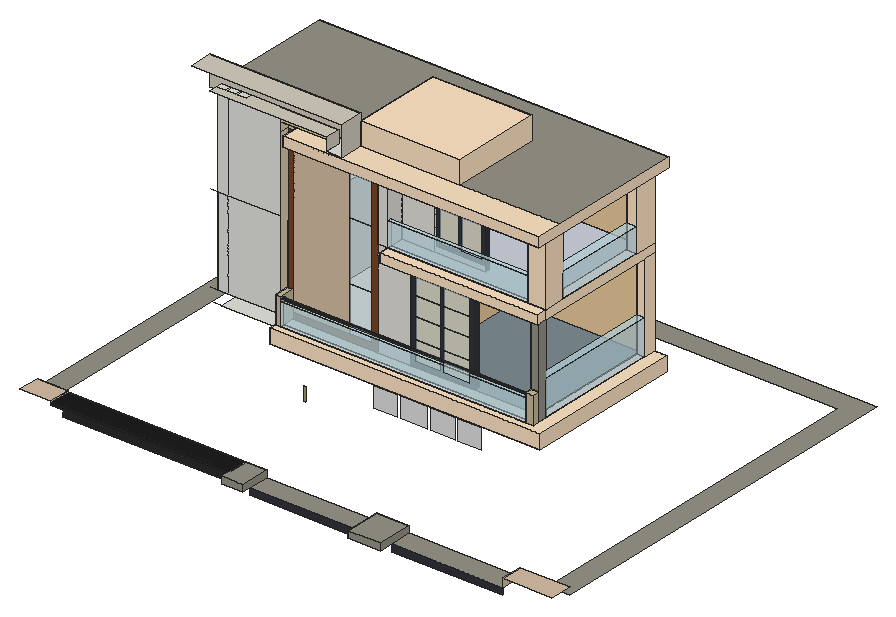
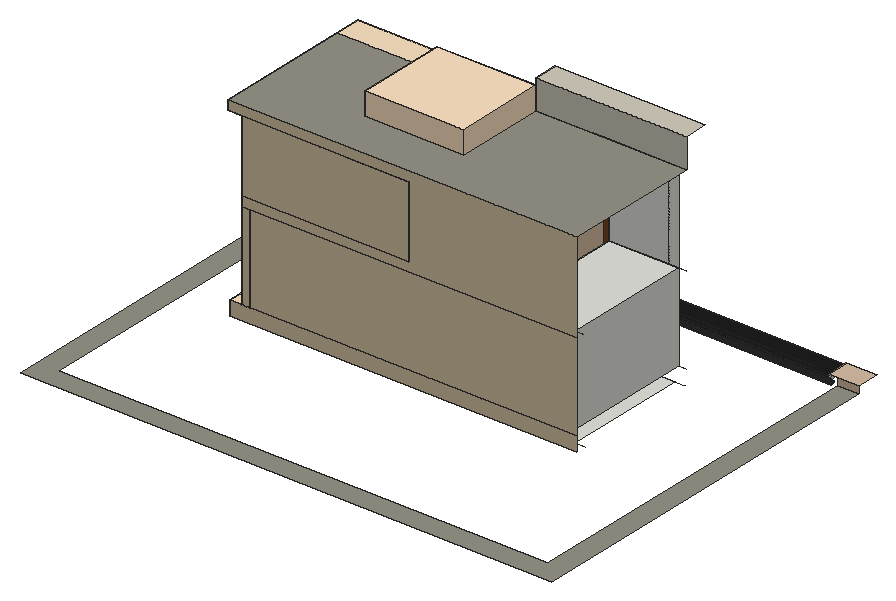
# SketchUp Ruby script. Lengths in inches.
U = 1.inch
M = Sketchup.active_model
def pt(a) = Geom::Point3d.new(a.map { |v| v * U })
def face(e, loops, mat)
  f = e.add_face(loops[0].map { |a| pt(a) })
  loops[1..].each { |l| e.add_face(l.map { |a| pt(a) }).erase! }
  f.material = f.back_material = mat if mat
  f
end
# faces: each face lists its corners as indices into pts; further lists are holes
def faces(e, pts, list, mat = nil) = list.each { |f| face(e, (f[0].is_a?(Array) ? f : [f]).map { |l| l.map { |i| pts[i] } }, mat) }
# xy, xz, yz: faces in a plane at the given z, y or x. An outline is a flat list of corners, or four numbers for a rectangle; further outlines are holes
def ring(l) = l.size == 4 ? [[l[0], l[1]], [l[2], l[1]], [l[2], l[3]], [l[0], l[3]]] : l.each_slice(2).to_a
def flat(e, list, mat, &to3) = list.each { |f| face(e, (f[0].is_a?(Array) ? f : [f]).map { |l| ring(l).map { |u, v| to3.(u, v) } }, mat) }
def xy(e, z, list, mat = nil) = flat(e, list, mat) { |x, y| [x, y, z] }
def xz(e, y, list, mat = nil) = flat(e, list, mat) { |x, z| [x, y, z] }
def yz(e, x, list, mat = nil) = flat(e, list, mat) { |y, z| [x, y, z] }
def lines(e, pts, list) = list.each { |a, b| e.add_line(pt(pts[a]), pt(pts[b])) }
# prism: a flat outline (further loops are holes) pulled along v
def prism(e, loops, v, mat = nil)
  f = face(e, loops, mat); d = Geom::Vector3d.new(v.map { |x| x * U })
  f.pushpull(f.normal.samedirection?(d) ? d.length : -d.length)
end
def box(e, o, s, mat = nil) = prism(e, [[o, [o[0] + s[0], o[1], o[2]], [o[0] + s[0], o[1] + s[1], o[2]], [o[0], o[1] + s[1], o[2]]]], [0, 0, s[2]], mat)
def at(x, y, z, deg = 0) = Geom::Transformation.translation(pt([x, y, z])) * Geom::Transformation.rotation(ORIGIN, Z_AXIS, deg.degrees)
def axes(o, x, y, z) = Geom::Transformation.new([*x, 0, *y, 0, *z, 0, *pt(o).to_a, 1])
def part(name) = M.definitions.add(name)
# library, detail: a bought-in or finely detailed component or shape, given as its bounding box
def library(name, o, s) = part(name).tap { |d| box(d.entities, o, s) }
def detail(e, o, s) = box(e.add_group.entities, o, s)
def put(e, d, t, mat = nil) = e.add_instance(d, t).tap { |i| i.material = mat if mat }
def group(e, t, mat = nil) = e.add_group.tap { |g| g.transformation = t; g.material = mat if mat }.entities
root = M.entities
M.materials.add("[0012_Bisque]").color = [252, 225, 194]
M.materials.add("[0012_Bisque]1").color = [255, 228, 196]
M.materials.add("[0035_Tan]").color = [234, 201, 156]
M.materials.add("[Color M08]").color = [30, 30, 30]
M.materials.add("[Concrete Pavers Block Multi]").color = [124, 140, 145]
M.materials.add("[Field Square Tile]").color = [217, 201, 169]
M.materials.add("[Formica Graystone]").color = [209, 204, 189]
M.materials.add("[Formica Graystone]1").color = [149, 146, 135]
M.materials.add("[Formica Laminate Dark]").color = [50, 53, 60]
M.materials.add("[Formica Laminate Light]").color = [213, 189, 164]
M.materials.add("[Marble Carrara Floor Tile]").color = [204, 208, 219]
M.materials.add("[Marble Carrara Gold Floor Tile]").color = [225, 223, 217]
M.materials.add("[Quartz Light Brown]").color = [199, 184, 152]
M.materials.add("[Translucent Glass Gray]").color = [128, 128, 128]
M.materials["[Translucent Glass Gray]"].alpha = 0.5
M.materials.add("[Translucent Glass Safety]").color = [204, 235, 244]
M.materials["[Translucent Glass Safety]"].alpha = 0.5
M.materials.add("[Wood Bamboo]").color = [177, 105, 43]
M.materials.add("[Wood Lumber ButtJoined]").color = [164, 152, 112]
M.materials.add("[Wood Veneer 01]").color = [120, 70, 37]
xy(root,70.6875,[[463.03,0,507.04,19.125],[284.59,8,312.84,19.125],[463.03,19.125,507.04,48.44]])
xy(root,70.6875,[[312.84,19.125,463.03,48.44],[507.04,19.125,658.96,48.44]],"[Formica Graystone]1")
xy(root,72,[[0,48.44,29.31,48.44,29.31,542.96,697.25,542.96,697.25,48.44,726.5625,48.44,726.5625,572.27,0,572.27]],"[Formica Graystone]1")
xy(root,76.75,[[153.57,19.125,161.5,27.41],[161.5,19.125,169.43,27.41],[41.54,27.41,48.35,37.79],[153.57,27.41,161.5,37.79],[161.5,27.41,169.43,37.79],
  [277.34,27.41,284.59,37.79],[153.57,37.79,161.5,48.44],[161.5,37.79,169.43,48.44]])
xy(root,76.75,[[41.54,19.125,41.54,27.41,48.35,27.41,48.35,37.79,41.54,37.79,41.54,48.44,153.57,48.44,153.57,19.125],[169.43,19.125,169.43,48.44,284.59,48.44,284.59,37.79,277.34,37.79,277.34,27.41,284.59,27.41,284.59,19.125]],"[Color M08]")
xy(root,79.91,[[41.54,19.125,284.59,48.44]],"[Color M08]")
xy(root,80,[[463.03,0,507.04,48.44],[284.59,8,312.84,48.44]],"[Formica Graystone]1")
xy(root,81.8125,[[0,19.125,41.54,48.44],[658.96,19.125,726.5625,48.44]],"[Formica Laminate Light]")
xy(root,118.13,[[320.36,216.4,477.43,230.18]])
xy(root,129,[[106.34,230.18,513.1,400.72],[513.1,230.18,526.89,414.5]])
xy(root,129,[[198.4375,197.31,567.07,216.4],[526.89,216.4,567.07,230.18],[526.89,230.18,567.07,414.5]],"[0012_Bisque]")
xy(root,148.25,[[198.4375,206.85,205.86,227.35],[205.86,206.85,539.81,211.77],[539.81,206.85,550.76,216.4],[205.86,211.77,539.81,227.35],[539.81,216.4,550.76,227.35],
  [103.52,227.35,198.4375,403.54],[198.4375,227.35,358.57,403.54],[358.57,227.35,367.31,403.54],[367.31,227.35,453.56,235.59],[539.81,227.35,550.76,396.98],
  [539.81,396.98,550.76,414.5]])
xy(root,148.25,[[198.4375,197.31,567.07,197.31,567.07,414.5,550.76,414.5,550.76,206.85,198.4375,206.85]],"[0012_Bisque]")
xy(root,148.25,[[453.56,227.35,539.81,227.35,539.81,403.54,367.31,403.54,367.31,235.59,453.56,235.59]],"[Concrete Pavers Block Multi]")
xy(root,178.125,[[205.86,206.85,539.81,211.77]],"[Translucent Glass Safety]")
xy(root,184.9375,[[198.4375,206.85,205.86,227.35],[539.81,206.85,550.76,216.4]],"[Quartz Light Brown]")
xy(root,196.25,[[539.81,227.35,550.76,396.98]],"[Translucent Glass Safety]")
xy(root,268.25,[[539.81,214.29,550.76,216.4],[539.81,216.4,550.76,227.35],[103.52,227.35,198.4375,403.54],[358.57,227.35,367.31,403.54],[367.31,227.35,453.56,235.59],
  [539.81,396.98,550.76,414.5],[198.4375,403.54,358.57,414.5],[358.57,403.54,367.31,414.5],[367.31,403.54,539.81,414.5]])
xy(root,268.25,[[335.01,214.29,539.81,227.35]],"[0012_Bisque]1")
xy(root,268.25,[[453.56,227.35,453.56,235.59,367.31,235.59,367.31,403.54,539.81,403.54,539.81,396.98,550.76,396.98,550.76,227.35]],"[Wood Bamboo]")
xy(root,280.9375,[[321.82,227.35,321.82,414.5,550.76,414.5,550.76,383,537.52,383,537.52,401.25,335.07,401.25,335.07,227.35],[335.07,227.35,526.35,233.16],[526.35,227.35,526.35,240.6,537.52,240.6,537.52,256.72,550.76,256.72,550.76,227.35],[335.07,251.53,449.88,256.72],[537.52,256.72,550.76,383]])
xy(root,280.9375,[[335.01,214.29,550.76,227.35]],"[0012_Bisque]1")
xy(root,280.9375,[[335.07,233.16,526.35,233.16,526.35,240.6,537.52,240.6,537.52,401.25,335.07,401.25,335.07,256.72,449.88,256.72,449.88,251.53,335.07,251.53]],"[Marble Carrara Floor Tile]")
xy(root,314.4375,[[335.07,227.35,526.35,233.16],[537.52,256.72,550.76,383]],"[Translucent Glass Safety]")
xy(root,379.375,[[321.82,227.35,321.82,414.5,550.76,414.5,550.76,383,537.52,383,537.52,401.25,335.07,401.25,335.07,227.35],[526.35,227.35,526.35,240.6,537.52,240.6,537.52,256.72,550.76,256.72,550.76,227.35],[335.07,251.53,449.88,256.72]])
xy(root,379.375,[[219.95,192.17,219.95,227.35,550.76,227.35,550.76,414.5,569.82,414.5,569.82,192.17]],"[0012_Bisque]1")
xy(root,379.375,[[335.07,227.35,335.07,251.53,449.88,251.53,449.88,256.72,335.07,256.72,335.07,401.25,537.52,401.25,537.52,383,550.76,383,550.76,256.72,537.52,256.72,537.52,240.6,526.35,240.6,526.35,227.35]],"[Wood Bamboo]")
xy(root,392.375,[[276.68,195.77,276.68,216.4,219.95,216.4,219.95,227.35,297.93,227.35,297.93,195.77],[198.4375,216.4,219.95,227.35],[297.93,227.35,433.12,350.92]])
xy(root,392.375,[[219.95,192.17,276.68,216.4],[276.68,192.17,297.93,195.77],[297.93,192.17,569.82,227.35]],"[0012_Bisque]")
xy(root,392.375,[[92.5625,227.35,297.93,227.35,297.93,350.92,433.12,350.92,433.12,227.35,569.82,227.35,569.82,414.5,92.5625,414.5]],"[Formica Graystone]1")
xy(root,409.95,[[117.23,208.71,128.74,216.4],[131.17,208.71,142.68,216.4],[145.54,208.71,157.05,216.4]])
xy(root,409.95,[[117.23,195.77,117.23,208.71,128.74,208.71,128.74,216.4,131.17,216.4,131.17,208.71,142.68,208.71,142.68,216.4,145.54,216.4,145.54,208.71,157.05,208.71,157.05,216.4,276.68,216.4,276.68,195.77]],"[Formica Graystone]")
xy(root,423.3125,[[297.93,227.35,433.12,350.92]],"[0012_Bisque]1")
xy(root,432.8125,[[92.5625,195.77,297.93,227.35]],"[Formica Graystone]")
xz(root,0,[[463.03,70.6875,507.04,80]],"[Formica Graystone]1")
xz(root,8,[[284.59,70.6875,312.84,80]],"[Formica Graystone]1")
xz(root,19.125,[[41.54,76.75,284.59,79.91]],"[Color M08]")
xz(root,19.125,[[507.04,61.39,658.96,70.6875],[312.84,61.83,463.03,70.6875]],"[Formica Laminate Dark]")
xz(root,48.44,[[41.54,76.75,284.59,79.91]],"[Color M08]")
xz(root,48.44,[[284.59,70.6875,312.84,80],[463.03,70.6875,507.04,80]],"[Formica Graystone]1")
xz(root,48.44,[[0,72,29.31,81.8125]],"[Formica Laminate Light]")
xz(root,192.17,[[219.95,379.375,569.82,392.375]],"[0012_Bisque]")
xz(root,197.31,[[198.4375,129,567.07,148.25]],"[0012_Bisque]")
xz(root,206.85,[[198.4375,148.25,205.86,184.9375],[539.81,148.25,550.76,184.9375]],"[Quartz Light Brown]")
xz(root,206.85,[[205.86,148.25,539.81,178.125]],"[Translucent Glass Safety]")
xz(root,211.77,[[205.86,148.25,539.81,178.125]],"[Translucent Glass Safety]")
xz(root,214.29,[[335.01,268.25,550.76,280.9375]],"[0012_Bisque]1")
xz(root,216.4,[[539.81,148.25,550.76,178.125],[539.81,178.125,550.76,184.9375]])
xz(root,216.4,[[198.4375,392.375,276.68,409.95]],"[Field Square Tile]")
xz(root,216.4,[[539.81,184.9375,550.76,268.25]],"[Formica Graystone]1")
xz(root,216.4,[[324.95,85.55,358.29,113.55],[361.76,85.55,398.73,113.55],[402.19,85.55,436.48,113.55],[439.94,85.55,472.85,113.55]],"[Translucent Glass Gray]")
xz(root,216.4,[[228.85,61.59,231.85,79.84]],"[Wood Lumber ButtJoined]")
xz(root,227.35,[[103.52,148.25,117.23,268.25],[117.23,148.25,198.4375,268.25],[198.4375,148.25,205.86,184.9375],[539.81,148.25,550.76,196.25],[103.52,268.25,117.23,392.375],
  [117.23,268.25,198.4375,392.375],[335.01,268.25,550.76,280.9375]])
xz(root,227.35,[[526.35,280.9375,550.76,379.375]],"[0012_Bisque]")
xz(root,227.35,[[297.93,392.375,433.12,423.3125]],"[0012_Bisque]1")
xz(root,227.35,[[198.4375,379.375,219.95,392.375]],"[Field Square Tile]")
xz(root,227.35,[[92.5625,392.375,297.93,432.8125]],"[Formica Graystone]")
xz(root,227.35,[[539.81,196.25,550.76,268.25]],"[Formica Graystone]1")
xz(root,227.35,[[[367.31,148.25,453.56,268.25],[373.52,154.46,447.35,262.04]],[407.96,154.46,412.12,262.04]],"[Formica Laminate Dark]")
xz(root,227.35,[[205.86,156.84,283.0625,156.84,283.0625,370.78,207.03,370.78,207.03,184.9375,205.86,184.9375]],"[Formica Laminate Light]")
xz(root,227.35,[[321.82,148.25,367.31,268.25],[321.82,268.25,335.01,280.9375],[321.82,280.9375,335.07,379.375]],"[Marble Carrara Gold Floor Tile]")
xz(root,227.35,[[373.52,154.46,407.96,182.08],[412.12,154.46,447.35,182.08],[283.0625,156.84,313.23,218.375],[373.52,182.08,407.96,209.7],[412.12,182.08,447.35,209.7],
  [373.52,209.7,407.96,236.15],[412.12,209.7,447.35,236.15],[283.0625,218.375,313.23,299.36],[373.52,236.15,407.96,262.04],[412.12,236.15,447.35,262.04],
  [335.07,280.9375,526.35,314.4375],[283.0625,299.36,313.23,370.78]],"[Translucent Glass Safety]")
xz(root,227.35,[[205.86,148.25,321.82,148.25,321.82,379.375,198.4375,379.375,198.4375,184.9375,207.03,184.9375,207.03,370.78,313.23,370.78,313.23,156.84,205.86,156.84]],"[Wood Veneer 01]")
xz(root,233.16,[[335.07,280.9375,526.35,314.4375]],"[Translucent Glass Safety]")
xz(root,235.59,[[367.31,148.25,453.56,268.25]],"[0035_Tan]")
xz(root,240.6,[[526.35,280.9375,537.52,379.375]],"[0012_Bisque]")
xz(root,251.53,[[[382.55,289.11,449.88,373.76],[387.45,294.01,444.98,368.86]],[413.33,294.01,417.3,368.86]],"[Formica Laminate Dark]")
xz(root,251.53,[[335.07,280.9375,380.32,379.375],[380.32,280.9375,449.88,280.9375,449.88,289.11,382.55,289.11,382.55,373.76,449.88,373.76,449.88,379.375,380.32,379.375]],"[Marble Carrara Gold Floor Tile]")
xz(root,251.53,[[387.45,294.01,413.33,368.86],[417.3,294.01,444.98,368.86]],"[Translucent Glass Safety]")
xz(root,256.72,[[537.52,280.9375,550.76,314.4375]])
xz(root,256.72,[[537.52,314.4375,550.76,379.375]],"[0012_Bisque]")
xz(root,256.72,[[335.07,280.9375,449.88,379.375]],"[0035_Tan]")
xz(root,350.92,[[297.93,392.375,433.12,423.3125]],"[0012_Bisque]1")
xz(root,383,[[537.52,280.9375,550.76,314.4375]])
xz(root,383,[[537.52,314.4375,550.76,379.375]],"[0012_Bisque]1")
xz(root,396.98,[[539.81,148.25,550.76,196.25]])
xz(root,396.98,[[539.81,196.25,550.76,268.25]],"[0012_Bisque]1")
xz(root,401.25,[[335.07,280.9375,537.52,379.375]],"[0035_Tan]")
xz(root,403.54,[[103.52,148.25,198.4375,268.25],[198.4375,148.25,358.57,268.25],[358.57,148.25,367.31,268.25]])
xz(root,403.54,[[367.31,148.25,539.81,268.25]],"[0035_Tan]")
xz(root,414.5,[[92.5625,129,567.07,148.25],[92.5625,148.25,539.81,268.25],[539.81,148.25,550.76,268.25],[92.5625,268.25,92.5625,392.375,569.82,392.375,569.82,379.375,321.82,379.375,321.82,280.9375,550.76,280.9375,550.76,268.25],[321.82,280.9375,550.76,379.375]],"[Field Square Tile]")
yz(root,41.54,[[19.125,76.75,48.44,79.91]])
yz(root,41.54,[[19.125,79.91,48.44,81.8125]],"[Formica Laminate Light]")
yz(root,48.35,[[33.0625,67.25,32.4,67.34,31.78,67.6,31.25,68,30.84,68.53,30.59,69.15,30.5,69.81,30.59,70.48,30.84,71.1,31.25,71.625,31.78,72.03,32.4,72.29,33.0625,72.38,33.73,72.29,34.34,72.03,34.875,71.625,35.28,71.1,35.54,70.48,35.625,69.81,35.54,69.15,35.28,68.53,34.875,68,34.34,67.6,33.73,67.34]])
yz(root,103.52,[[227.35,148.25,403.54,268.25]])
yz(root,198.4375,[[216.4,148.25,227.35,184.9375],[227.35,148.25,403.54,268.25]])
yz(root,198.4375,[[197.31,129,216.4,148.25]],"[0012_Bisque]")
yz(root,198.4375,[[216.4,184.9375,227.35,379.375],[216.4,379.375,227.35,392.375]],"[Field Square Tile]")
yz(root,198.4375,[[206.85,148.25,216.4,184.9375]],"[Quartz Light Brown]")
yz(root,205.86,[[206.85,148.25,211.77,178.125],[209.66,180.85,209.4,180.88,209.16,180.98,208.95,181.14,208.79,181.35,208.69,181.59,208.66,181.85,208.69,182.11,208.79,182.35,208.95,182.55,209.16,182.71,209.4,182.8125,209.66,182.85,209.91,182.8125,210.16,182.71,210.36,182.55,210.52,182.35,210.62,182.11,210.66,181.85,210.62,181.59,210.52,181.35,210.36,181.14,210.16,180.98,209.91,180.88]])
yz(root,205.86,[[[211.77,148.25,227.35,148.25,227.35,184.9375,206.85,184.9375,206.85,178.125,211.77,178.125],[209.66,180.85,209.4,180.88,209.16,180.98,208.95,181.14,208.79,181.35,208.69,181.59,208.66,181.85,208.69,182.11,208.79,182.35,208.95,182.55,209.16,182.71,209.4,182.8125,209.66,182.85,209.91,182.8125,210.16,182.71,210.36,182.55,210.52,182.35,210.62,182.11,210.66,181.85,210.62,181.59,210.52,181.35,210.36,181.14,210.16,180.98,209.91,180.88]]],"[Quartz Light Brown]")
yz(root,219.95,[[192.17,379.375,227.35,392.375]],"[0012_Bisque]")
yz(root,276.68,[[195.77,392.375,216.4,409.95]],"[Formica Graystone]")
yz(root,284.59,[[19.125,76.75,48.44,79.91]])
yz(root,297.93,[[227.35,392.375,350.92,423.3125]],"[0012_Bisque]1")
yz(root,297.93,[[195.77,392.375,227.35,432.8125]],"[Formica Graystone]")
yz(root,312.84,[[8,70.6875,48.44,80]],"[Formica Graystone]1")
yz(root,321.82,[[227.35,280.9375,414.5,379.375]])
yz(root,335.01,[[214.29,268.25,227.35,280.9375]],"[0012_Bisque]1")
yz(root,335.07,[[227.35,280.9375,233.16,314.4375],[251.53,280.9375,256.72,379.375]])
yz(root,335.07,[[256.72,280.9375,401.25,379.375]],"[0035_Tan]")
yz(root,335.07,[[233.16,280.9375,251.53,280.9375,251.53,379.375,227.35,379.375,227.35,314.4375,233.16,314.4375]],"[Marble Carrara Gold Floor Tile]")
yz(root,367.31,[[227.35,148.25,235.59,268.25]])
yz(root,367.31,[[235.59,148.25,403.54,268.25]],"[0035_Tan]")
yz(root,433.12,[[227.35,392.375,350.92,423.3125]],"[0012_Bisque]1")
yz(root,449.88,[[251.53,280.9375,256.72,379.375]],"[Formica Laminate Dark]")
yz(root,453.56,[[227.35,148.25,235.59,268.25]],"[Formica Laminate Dark]")
yz(root,463.03,[[0,70.6875,48.44,80]],"[Formica Graystone]1")
yz(root,507.04,[[0,70.6875,48.44,80]],"[Formica Graystone]1")
yz(root,526.35,[[227.35,280.9375,233.16,314.4375],[233.16,280.9375,240.6,314.4375]])
yz(root,526.35,[[227.35,314.4375,240.6,379.375]],"[0012_Bisque]")
yz(root,537.52,[[240.6,280.9375,256.72,379.375]],"[0012_Bisque]")
yz(root,537.52,[[383,280.9375,401.25,379.375]],"[0012_Bisque]1")
yz(root,537.52,[[256.72,280.9375,383,314.4375]],"[Translucent Glass Safety]")
yz(root,539.81,[[206.85,148.25,211.77,178.125],[211.77,148.25,216.4,178.125],[403.54,148.25,414.5,268.25]])
yz(root,539.81,[[396.98,148.25,403.54,268.25]],"[0012_Bisque]1")
yz(root,539.81,[[216.4,148.25,227.35,268.25]],"[Formica Graystone]1")
yz(root,539.81,[[[206.85,178.125,211.77,184.9375],[209.66,180.85,209.91,180.88,210.16,180.98,210.36,181.14,210.52,181.35,210.62,181.59,210.66,181.85,210.62,182.11,210.52,182.35,210.36,182.55,210.16,182.71,209.91,182.8125,209.66,182.85,209.4,182.8125,209.16,182.71,208.95,182.55,208.79,182.35,208.69,182.11,208.66,181.85,208.69,181.59,208.79,181.35,208.95,181.14,209.16,180.98,209.4,180.88]],[211.77,178.125,216.4,184.9375]],"[Quartz Light Brown]")
yz(root,539.81,[[227.35,148.25,396.98,196.25]],"[Translucent Glass Safety]")
yz(root,550.76,[[227.35,280.9375,256.72,379.375]],"[0012_Bisque]")
yz(root,550.76,[[396.98,148.25,414.5,268.25],[214.29,268.25,227.35,280.9375],[227.35,268.25,414.5,280.9375],[383,280.9375,414.5,379.375]],"[0012_Bisque]1")
yz(root,550.76,[[216.4,148.25,227.35,268.25]],"[Formica Graystone]1")
yz(root,550.76,[[206.85,148.25,216.4,184.9375]],"[Quartz Light Brown]")
yz(root,550.76,[[227.35,148.25,396.98,196.25],[256.72,280.9375,383,314.4375]],"[Translucent Glass Safety]")
yz(root,567.07,[[197.31,129,414.5,148.25]],"[0012_Bisque]")
yz(root,569.82,[[192.17,379.375,414.5,392.375]],"[0012_Bisque]")
yz(root,658.96,[[19.125,70.6875,48.44,81.8125]],"[Formica Laminate Light]")
p = [[48.35,30.59,60.84],[48.35,30.84,60.22],[277.34,30.84,60.22],[277.34,30.59,60.84],[48.35,35.28,60.22],[48.35,35.54,60.84],
  [277.34,35.54,60.84],[277.34,35.28,60.22],[48.35,30.5,61.5],[277.34,30.5,61.5],[48.35,35.625,61.5],[277.34,35.625,61.5],
  [48.35,30.59,62.17],[277.34,30.59,62.17],[48.35,35.54,62.17],[277.34,35.54,62.17],[48.35,30.84,62.78],[277.34,30.84,62.78],
  [48.35,35.28,62.78],[277.34,35.28,62.78],[48.35,31.25,63.3125],[277.34,31.25,63.3125],[48.35,34.875,63.3125],[277.34,34.875,63.3125],
  [48.35,31.78,63.72],[277.34,31.78,63.72],[48.35,34.34,63.72],[277.34,34.34,63.72],[48.35,32.4,63.98],[277.34,32.4,63.98],
  [48.35,33.73,63.98],[277.34,33.73,63.98],[48.35,33.0625,64.06],[277.34,33.0625,64.06],[48.35,31.78,67.6],[48.35,32.4,67.34],
  [277.34,32.4,67.34],[277.34,31.78,67.6],[48.35,33.0625,67.25],[277.34,33.0625,67.25],[48.35,33.73,67.34],[277.34,33.73,67.34],
  [48.35,34.34,67.6],[277.34,34.34,67.6],[48.35,31.25,68],[277.34,31.25,68],[48.35,34.875,68],[277.34,34.875,68],
  [48.35,30.84,68.53],[277.34,30.84,68.53],[48.35,35.28,68.53],[277.34,35.28,68.53],[48.35,30.59,69.15],[277.34,30.59,69.15],
  [48.35,35.54,69.15],[277.34,35.54,69.15],[48.35,30.5,69.81],[277.34,30.5,69.81],[48.35,35.625,69.81],[277.34,35.625,69.81],
  [48.35,30.59,70.48],[277.34,30.59,70.48],[48.35,35.54,70.48],[277.34,35.54,70.48],[48.35,30.84,71.1],[277.34,30.84,71.1],
  [48.35,35.28,71.1],[277.34,35.28,71.1],[48.35,31.25,71.625],[277.34,31.25,71.625],[48.35,34.875,71.625],[277.34,34.875,71.625],
  [48.35,31.78,72.03],[277.34,31.78,72.03],[48.35,34.34,72.03],[277.34,34.34,72.03],[48.35,32.4,72.29],[277.34,32.4,72.29],
  [48.35,33.73,72.29],[277.34,33.73,72.29],[48.35,33.0625,72.38],[277.34,33.0625,72.38],[205.86,209.4,180.88],[205.86,209.66,180.85],
  [539.81,209.66,180.85],[539.81,209.4,180.88],[205.86,209.91,180.88],[539.81,209.91,180.88],[205.86,209.16,180.98],[539.81,209.16,180.98],
  [205.86,210.16,180.98],[539.81,210.16,180.98],[205.86,208.95,181.14],[539.81,208.95,181.14],[205.86,210.36,181.14],[539.81,210.36,181.14],
  [205.86,208.79,181.35],[539.81,208.79,181.35],[205.86,210.52,181.35],[539.81,210.52,181.35],[205.86,208.69,181.59],[539.81,208.69,181.59],
  [205.86,210.62,181.59],[539.81,210.62,181.59],[205.86,208.66,181.85],[539.81,208.66,181.85],[205.86,210.66,181.85],[539.81,210.66,181.85],
  [205.86,208.69,182.11],[539.81,208.69,182.11],[205.86,210.62,182.11],[539.81,210.62,182.11],[205.86,208.79,182.35],[539.81,208.79,182.35],
  [205.86,210.52,182.35],[539.81,210.52,182.35],[205.86,208.95,182.55],[539.81,208.95,182.55],[205.86,210.36,182.55],[539.81,210.36,182.55],
  [205.86,209.16,182.71],[539.81,209.16,182.71],[205.86,210.16,182.71],[539.81,210.16,182.71],[205.86,209.4,182.8125],[539.81,209.4,182.8125],
  [205.86,209.91,182.8125],[539.81,209.91,182.8125],[205.86,209.66,182.85],[539.81,209.66,182.85],[106.34,230.18,129],[92.5625,230.18,129],
  [106.34,400.72,129],[92.5625,400.72,129],[103.52,227.35,148.25],[92.5625,227.35,148.25],[103.52,227.35,268.25],[92.5625,227.35,268.25],
  [103.52,403.54,268.25],[92.5625,403.54,268.25]]
faces(root,p,[[0,1,2,3],[4,5,6,7],[8,0,3,9],[5,10,11,6],[12,8,9,13],[10,14,15,11],[16,12,13,17],[14,18,19,15],
  [20,16,17,21],[18,22,23,19],[24,20,21,25],[22,26,27,23],[28,24,25,29],[26,30,31,27],[32,28,29,33],[30,32,33,31],
  [34,35,36,37],[35,38,39,36],[38,40,41,39],[40,42,43,41],[44,34,37,45],[42,46,47,43],[48,44,45,49],[46,50,51,47],
  [52,48,49,53],[50,54,55,51],[56,52,53,57],[54,58,59,55],[60,56,57,61],[58,62,63,59],[64,60,61,65],[62,66,67,63],
  [68,64,65,69],[66,70,71,67],[72,68,69,73],[70,74,75,71],[76,72,73,77],[74,78,79,75],[80,76,77,81],[78,80,81,79]],"[Formica Laminate Dark]")
faces(root,p,[[82,83,84,85],[83,86,87,84],[88,82,85,89],[86,90,91,87],[92,88,89,93],[90,94,95,91],[96,92,93,97],[94,98,99,95],
  [100,96,97,101],[98,102,103,99],[104,100,101,105],[102,106,107,103],[108,104,105,109],[106,110,111,107],[112,108,109,113],[110,114,115,111],
  [116,112,113,117],[114,118,119,115],[120,116,117,121],[118,122,123,119],[124,120,121,125],[122,126,127,123],[128,124,125,129],[126,128,129,127]],"[Formica Graystone]")
lines(root,p,[[130,131],[132,133],[134,135],[136,137],[138,139]])
